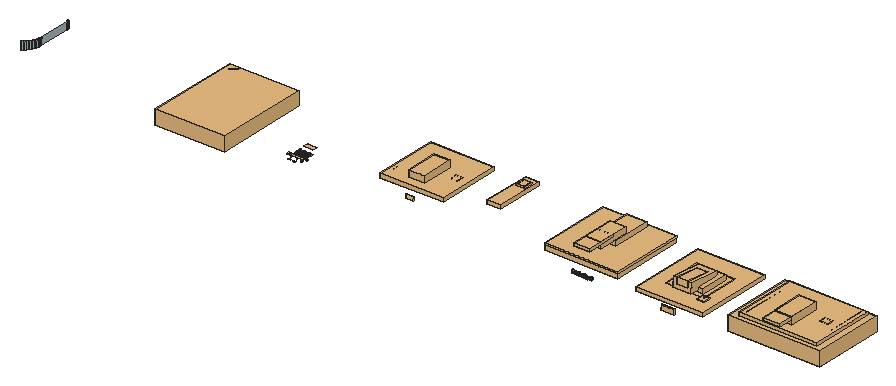
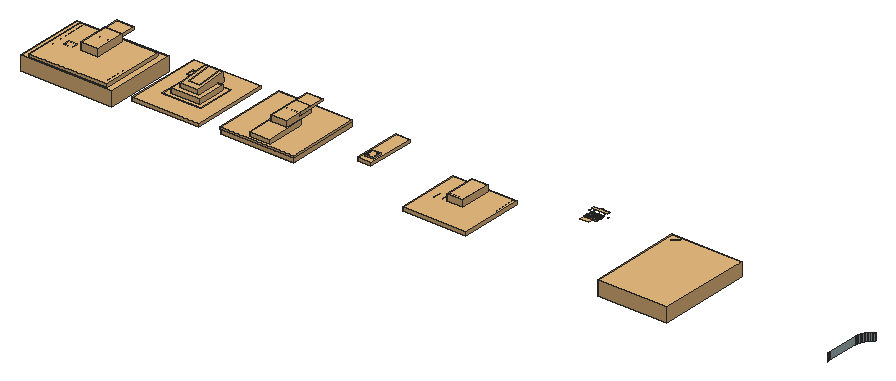
# SketchUp Ruby script. Lengths in inches.
U = 1.inch
M = Sketchup.active_model
def pt(a) = Geom::Point3d.new(a.map { |v| v * U })
def face(e, loops, mat)
  f = e.add_face(loops[0].map { |a| pt(a) })
  loops[1..].each { |l| e.add_face(l.map { |a| pt(a) }).erase! }
  f.material = f.back_material = mat if mat
  f
end
# faces: each face lists its corners as indices into pts; further lists are holes
def faces(e, pts, list, mat = nil) = list.each { |f| face(e, (f[0].is_a?(Array) ? f : [f]).map { |l| l.map { |i| pts[i] } }, mat) }
# xy, xz, yz: faces in a plane at the given z, y or x. An outline is a flat list of corners, or four numbers for a rectangle; further outlines are holes
def ring(l) = l.size == 4 ? [[l[0], l[1]], [l[2], l[1]], [l[2], l[3]], [l[0], l[3]]] : l.each_slice(2).to_a
def flat(e, list, mat, &to3) = list.each { |f| face(e, (f[0].is_a?(Array) ? f : [f]).map { |l| ring(l).map { |u, v| to3.(u, v) } }, mat) }
def xy(e, z, list, mat = nil) = flat(e, list, mat) { |x, y| [x, y, z] }
def xz(e, y, list, mat = nil) = flat(e, list, mat) { |x, z| [x, y, z] }
def yz(e, x, list, mat = nil) = flat(e, list, mat) { |y, z| [x, y, z] }
def lines(e, pts, list) = list.each { |a, b| e.add_line(pt(pts[a]), pt(pts[b])) }
# prism: a flat outline (further loops are holes) pulled along v
def prism(e, loops, v, mat = nil)
  f = face(e, loops, mat); d = Geom::Vector3d.new(v.map { |x| x * U })
  f.pushpull(f.normal.samedirection?(d) ? d.length : -d.length)
end
def box(e, o, s, mat = nil) = prism(e, [[o, [o[0] + s[0], o[1], o[2]], [o[0] + s[0], o[1] + s[1], o[2]], [o[0], o[1] + s[1], o[2]]]], [0, 0, s[2]], mat)
def at(x, y, z, deg = 0) = Geom::Transformation.translation(pt([x, y, z])) * Geom::Transformation.rotation(ORIGIN, Z_AXIS, deg.degrees)
def axes(o, x, y, z) = Geom::Transformation.new([*x, 0, *y, 0, *z, 0, *pt(o).to_a, 1])
def part(name) = M.definitions.add(name)
# library, detail: a bought-in or finely detailed component or shape, given as its bounding box
def library(name, o, s) = part(name).tap { |d| box(d.entities, o, s) }
def detail(e, o, s) = box(e.add_group.entities, o, s)
def put(e, d, t, mat = nil) = e.add_instance(d, t).tap { |i| i.material = mat if mat }
def group(e, t, mat = nil) = e.add_group.tap { |g| g.transformation = t; g.material = mat if mat }.entities
root = M.entities
M.materials.add("1").color = [0, 0, 0]
M.materials.add("11").color = [255, 255, 255]
M.materials.add("12").color = [5, 5, 5]
M.materials.add("2").color = [12, 12, 16]
M.materials.add("24").color = [74, 74, 74]
M.materials.add("26").color = [169, 186, 191]
M.materials.add("8").color = [50, 50, 50]
M.materials.add("9").color = [44, 44, 44]
c1 = library("Group89",[-140.11,-176.26,170.27],[282.52,381.26,57.85])
c2 = library("Group78",[38808.2,7300.17,1634.6875],[7.14,3.55,0.08])
c3 = library("Group72",[38808.13,7304.67,1634.69],[7.28,3.54,0.08])
c4 = library("Group73",[38807.56,7322.91,1634.71],[8.42,4.13,0.08])
c5 = library("om.cn_51",[-14089.91,-120000,166752.75],[16176.5,10000,4589.03])
c6 = library("om.cn_51698238",[-12277.97,-120000,175247.47],[24687.75,10000,11950.5])
c7 = library("Group79",[38826.73,7301.99,1634.69],[8.28,4.18,0.08])
c8 = library("Group74",[38826.7,7322.86,1634.71],[8.34,4.15,0.08])
c9 = library("om.cn_51268574",[-7425.4375,-120000,166763.1875],[21515.3125,10000,4564.15])
c10 = library("Group80",[38845.76,7302.01,1634.69],[8.44,4.16,0.08])
c11 = library("Group76",[38845.73,7322.86,1634.71],[8.5,4.18,0.08])
c12 = library("om.cn_32",[-31.33,-200.31,17.07],[62.68,126.37,27.34])
c13 = library("om.cn_32430148",[-31.33,-200.31,34.56],[62.68,118.17,8.93])
c14 = library("Group41",[2.42,129.72,-129.67],[259.34,15.26,259.34])
c15 = library("Group42",[13.39,138.09,-118.66],[237.39,3.26,237.32])
c16 = library("Group39",[-54.28,-6.65,-0.51],[57.5,23.32,1.99])
c17 = library("Group43",[197.75,140.28,-13.26],[27.5,3.46,26.52])
c18 = library("Group30",[-30.87,-113.18,-1.53],[61.73,214.81,14.15])
c19 = library("Group35",[-24.97,-25.2,0],[49.93,50.08,7.81])
c20 = library("Group16",[-41.15,-138.36,2.25],[82.3,160.65,19.68])
c21 = library("Group14",[-159,-159,0.16],[318,318,8.06])
c22 = library("Group13",[-149.91,-149.91,254.4375],[299.82,299.82,15.58])
c23 = library("Group46",[60.41,189.4,-65.28],[131.43,26.74,130.56])
c24 = library("Group53",[39.65,186.43,-85.24],[172.95,8.17,170.48])
c25 = library("Group54",[-24.48,177.31,-174.76],[301.22,16.77,349.52])
c26 = library("Group49",[134.43,190.47,6.48],[47.92,30.54,112.32])
c27 = library("Group55",[117.125,172.9375,-23.28],[82.52,48.07,142.08])
c28 = library("Group52",[-54.25,-6.65,-1.45],[57.46,23.32,2.82])
c29 = library("Group51",[197.5,187.71,76.61],[33.96,7.14,33.51])
c30 = library("Group5",[-32.86,-200.31,17.11],[65.72,126.37,27.3])
c31 = library("Group6",[-32.49,-200.31,34.57],[64.98,118.17,8.93])
c32 = library("Group7",[-18.29,129.75,-129.67],[300.75,15.26,259.34])
c33 = library("Group",[-44.84,79.83,-140.46],[353.86,54.36,289.99])
c34 = library("Group8",[40587.56,7377.77,1637.51],[284.38,237.38,4.11])
c35 = library("Group10",[40712.23,7354.21,1598.9],[39.27,4.15,12.57])
c36 = library("Group9",[206.09,140.95,-13.26],[31.34,3.18,26.52])
xy(root,91.8361,[[298.2685,7.251,298.2737,7.2799,298.2785,7.3089],[298.2785,7.3089,298.2831,7.3379,298.2873,7.367],[298.2873,7.367,298.2914,7.3965,298.2951,7.426],[298.2951,7.426,298.2985,7.4555,298.3017,7.4851],[298.3017,7.4851,298.3045,7.5147,298.3071,7.5443],
  [298.3092,12.9012,298.3071,12.9296,298.3045,12.9592],[298.3045,12.9592,298.3017,12.9888,298.2985,13.0184,298.2914,13.0775],[298.2985,13.0184,298.2951,13.048,298.2914,13.0775],[298.2914,13.0775,298.2873,13.107,298.2831,13.136]],"26")
xy(root,92.317,[[[384.7707,4.8659,390.0066,4.8659,390.2382,4.874,390.2707,4.8765,390.3033,4.8793,390.3357,4.8824,390.3682,4.8858,390.4006,4.8896,390.433,4.8937,390.4654,4.8981,390.4973,4.9028,390.5291,4.9078,390.5609,4.9131,390.5927,4.9188,390.6244,4.9248,390.656,4.931,390.6876,4.9376,390.9044,4.9919,391.1152,5.0606,391.3194,5.1429,391.5165,5.2385,391.7059,5.3467,391.8871,5.4669,392.0595,5.5987,392.2226,5.7415,392.3758,5.8947,392.5186,6.0578,392.6504,6.2302,392.7707,6.4114,392.8788,6.6008,392.9744,6.7979,393.0568,7.0021,393.1254,7.2129,393.1797,7.4297,393.1863,7.4613,393.1926,7.4929,393.1985,7.5246,393.2042,7.5564,393.2095,7.5882,393.2145,7.6201,393.2192,7.652,393.2236,7.6843,393.2277,7.7167,393.2315,7.7491,393.2349,7.7816,393.2381,7.8141,393.2408,7.8466,393.2433,7.8791,393.2515,8.1107,393.2515,13.3466,393.2433,13.5782,393.2408,13.6107,393.2381,13.6432,393.2349,13.6757,393.2315,13.7082,393.2277,13.7406,393.2236,13.773,393.2192,13.8053,393.2145,13.8372,393.2095,13.8691,393.2042,13.9009,393.1985,13.9327,393.1926,13.9644,393.1863,13.996,393.1797,14.0276,393.1254,14.2444,393.0568,14.4552,392.9744,14.6594,392.8788,14.8565,392.7707,15.0459,392.6504,15.2271,392.5186,15.3995,392.3758,15.5626,392.2226,15.7158,392.0595,15.8586,391.8871,15.9904,391.7059,16.1106,391.5165,16.2188,391.3194,16.3144,391.1152,16.3967,390.9044,16.4654,390.6876,16.5197,390.656,16.5263,390.6244,16.5326,390.5927,16.5385,390.5609,16.5442,390.5291,16.5495,390.4973,16.5545,390.4654,16.5592,390.433,16.5636,390.4006,16.5677,390.3682,16.5715,390.3357,16.5749,390.3033,16.578,390.2707,16.5808,390.2382,16.5833,390.0066,16.5914,384.7707,16.5914,384.5392,16.5833,384.5066,16.5808,384.4741,16.578,384.4416,16.5749,384.4091,16.5715,384.3767,16.5677,384.3443,16.5636,384.312,16.5592,384.2801,16.5545,384.2482,16.5495,384.2164,16.5442,384.1846,16.5385,384.1529,16.5326,384.1213,16.5263,384.0897,16.5197,383.8729,16.4654,383.6622,16.3967,383.458,16.3144,383.2609,16.2188,383.0715,16.1106,382.8903,15.9904,382.7178,15.8586,382.5548,15.7158,382.4015,15.5626,382.2588,15.3995,382.127,15.2271,382.0067,15.0459,381.8985,14.8565,381.803,14.6594,381.7206,14.4552,381.652,14.2444,381.5976,14.0276,381.5911,13.996,381.5848,13.9644,381.5788,13.9327,381.5732,13.9009,381.5678,13.8691,381.5628,13.8372,381.5581,13.8053,381.5537,13.773,381.5496,13.7406,381.5459,13.7082,381.5424,13.6757,381.5393,13.6432,381.5365,13.6107,381.534,13.5782,381.5259,13.3466,381.5259,8.1107,381.534,7.8791,381.5365,7.8466,381.5393,7.8141,381.5424,7.7816,381.5459,7.7491,381.5496,7.7167,381.5537,7.6843,381.5581,7.652,381.5628,7.6201,381.5678,7.5882,381.5732,7.5564,381.5788,7.5246,381.5848,7.4929,381.591,7.4613,381.5976,7.4297,381.652,7.2129,381.7206,7.0021,381.803,6.7979,381.8985,6.6008,382.0067,6.4114,382.127,6.2302,382.2588,6.0578,382.4015,5.8947,382.5548,5.7415,382.7178,5.5987,382.8903,5.4669,383.0714,5.3467,383.2609,5.2385,383.4579,5.1429,383.6622,5.0606,383.8729,4.9919,384.0897,4.9376,384.1213,4.931,384.1529,4.9248,384.1846,4.9188,384.2164,4.9131,384.2482,4.9078,384.2801,4.9028,384.312,4.8981,384.3443,4.8937,384.3767,4.8896,384.4091,4.8858,384.4416,4.8824,384.4741,4.8793,384.5066,4.8765,384.5392,4.874],[381.6833,7.4494,381.6772,7.4788,381.6711,7.5096,381.6653,7.5404,381.6598,7.5713,381.6498,7.6333,381.6452,7.6643,381.6409,7.6958,381.6369,7.7273,381.6332,7.7588,381.6299,7.7904,381.6269,7.822,381.6241,7.8537,381.6218,7.884,381.6269,7.822,381.6409,7.6958,381.6598,7.5713,381.6711,7.5096],[393.1555,13.5733,393.1505,13.6353,393.1364,13.7615,393.1175,13.886,393.1062,13.9477,393.094,14.0079,393.1001,13.9785,393.1062,13.9477,393.112,13.9169,393.1175,13.886,393.1276,13.824,393.1321,13.793,393.1364,13.7615,393.1404,13.73,393.1441,13.6985,393.1475,13.6669,393.1505,13.6353,393.1532,13.6036],[384.1094,16.434,384.1388,16.4401,384.1696,16.4462,384.2005,16.452,384.2314,16.4575,384.2933,16.4676,384.3243,16.4721,384.3558,16.4764,384.3873,16.4804,384.4189,16.4841,384.4504,16.4874,384.4821,16.4905,384.5137,16.4932,384.544,16.4955,384.4821,16.4905,384.3558,16.4764,384.2314,16.4575,384.1696,16.4462],[390.2333,4.9618,390.2953,4.9668,390.4216,4.9809,390.546,4.9998,390.6077,5.0111,390.6679,5.0233,390.6385,5.0172,390.6077,5.0111,390.5769,5.0053,390.546,4.9998,390.4841,4.9897,390.453,4.9852,390.4216,4.9809,390.39,4.9769,390.3585,4.9732,390.3269,4.9699,390.2953,4.9668,390.2637,4.9641],[393.112,7.5404,393.1227,7.6023,393.1321,7.6643,393.1404,7.7273,393.1475,7.7904,393.1532,7.8537,393.1505,7.822,393.1475,7.7904,393.1441,7.7588,393.1404,7.7273,393.1364,7.6958,393.1321,7.6643,393.1276,7.6333,393.1227,7.6023,393.1175,7.5713],[381.6241,13.6036,381.6269,13.6353,381.6299,13.6669,381.6332,13.6985,381.6369,13.73,381.6409,13.7615,381.6452,13.793,381.6498,13.824,381.6546,13.855,381.6598,13.886,381.6653,13.9169,381.6546,13.855,381.6452,13.793,381.6369,13.73,381.6299,13.6669],[390.5769,16.452,390.515,16.4627,390.453,16.4721,390.39,16.4804,390.3269,16.4874,390.2637,16.4932,390.2953,16.4905,390.3269,16.4874,390.3585,16.4841,390.39,16.4804,390.4216,16.4764,390.453,16.4721,390.4841,16.4676,390.515,16.4627,390.546,16.4575],[384.5137,4.9641,384.4821,4.9668,384.4504,4.9699,384.4189,4.9732,384.3873,4.9769,384.3558,4.9809,384.3243,4.9852,384.2933,4.9897,384.2623,4.9946,384.2314,4.9998,384.2005,5.0053,384.2623,4.9946,384.3243,4.9852,384.3873,4.9769,384.4504,4.9699]],[390.2333,4.9618,390.2637,4.9641,390.2953,4.9668],[384.5137,4.9641,384.4504,4.9699,384.4821,4.9668],[390.2953,4.9668,390.3269,4.9699,390.3585,4.9732,390.4216,4.9809],[384.4504,4.9699,384.3873,4.9769,384.4189,4.9732],
  [390.3585,4.9732,390.39,4.9769,390.4216,4.9809],[384.3873,4.9769,384.3243,4.9852,384.3558,4.9809],[390.4216,4.9809,390.453,4.9852,390.4841,4.9897],[390.4216,4.9809,390.4841,4.9897,390.546,4.9998],[384.3243,4.9852,384.2623,4.9946,384.2933,4.9897],
  [384.2623,4.9946,384.2005,5.0053,384.2314,4.9998],[390.546,4.9998,390.5769,5.0053,390.6077,5.0111],[390.6077,5.0111,390.6385,5.0172,390.6679,5.0233],[381.6833,7.4494,381.6711,7.5096,381.6772,7.4788],[381.6711,7.5096,381.6598,7.5713,381.6653,7.5404],
  [393.112,7.5404,393.1175,7.5713,393.1227,7.6023],[381.6598,7.5713,381.6409,7.6958,381.6498,7.6333],[393.1227,7.6023,393.1276,7.6333,393.1321,7.6643],[381.6498,7.6333,381.6409,7.6958,381.6452,7.6643],[393.1321,7.6643,393.1364,7.6958,393.1404,7.7273],
  [381.6409,7.6958,381.6269,7.822,381.6299,7.7904,381.6332,7.7588],[381.6409,7.6958,381.6332,7.7588,381.6369,7.7273],[393.1404,7.7273,393.1441,7.7588,393.1475,7.7904],[393.1475,7.7904,393.1505,7.822,393.1532,7.8537],[381.6269,7.822,381.6218,7.884,381.6241,7.8537]],"8")
yz(root,298.3991,[[7.7851,90.6622,12.6889,91.8361]],"26")
p = [[297.1213,5.309,90.6622],[297.1213,5.309,91.8361],[296.9516,5.1964,91.8361],[296.9516,5.1964,90.6622],[297.2827,5.4324,90.6622],[297.2827,5.4324,91.8361],
  [297.4355,5.5662,90.6622],[297.4355,5.5662,91.8361],[297.579,5.7097,90.6622],[297.579,5.7097,91.8361],[297.7127,5.8624,90.6622],[297.7127,5.8624,91.8361],
  [297.8361,6.0239,90.6622],[297.8361,6.0239,91.8361],[297.9488,6.1936,90.6622],[297.9488,6.1936,91.8361],[298.0501,6.371,90.6622],[298.0501,6.371,91.8361],
  [298.1396,6.5556,90.6622],[298.1396,6.5556,91.8361],[298.2167,6.7468,90.6622],[298.2167,6.7468,91.8361],[298.281,6.9442,90.6622],[298.281,6.9442,91.8361],
  [298.3319,7.1473,90.6622],[298.3319,7.1473,91.8361],[298.3381,7.1768,90.6622],[298.3381,7.1768,91.8361],[298.3439,7.2065,90.6622],[298.3439,7.2065,91.8361],
  [298.3495,7.2362,90.6622],[298.3495,7.2362,91.8361],[298.3548,7.2659,90.6622],[298.3548,7.2659,91.8361],[298.3598,7.2957,90.6622],[298.3598,7.2957,91.8361],
  [298.3645,7.3255,90.6622],[298.3645,7.3255,91.8361],[298.3689,7.3554,90.6622],[298.3689,7.3554,91.8361],[298.373,7.3857,90.6622],[298.373,7.3857,91.8361],
  [298.3768,7.4161,90.6622],[298.3768,7.4161,91.8361],[298.3804,7.4464,90.6622],[298.3804,7.4464,91.8361],[298.3836,7.4768,90.6622],[298.3836,7.4768,91.8361],
  [298.3865,7.5073,90.6622],[298.3865,7.5073,91.8361],[298.3891,7.5377,90.6622],[298.3891,7.5377,91.8361],[298.3914,7.5682,90.6622],[298.3914,7.5682,91.8361],
  [298.3991,7.7851,90.6622],[298.3991,7.7851,91.8361],[298.3915,12.9057,90.6622],[298.3915,12.9057,91.8361],[298.3991,12.6889,91.8361],[298.3991,12.6889,90.6622],
  [298.3865,12.9667,90.6622],[298.3865,12.9667,91.8361],[298.3891,12.9362,91.8361],[298.3891,12.9362,90.6622],[298.3768,13.0579,90.6622],[298.3768,13.0579,91.8361],
  [298.3804,13.0275,91.8361],[298.3804,13.0275,90.6622],[298.3836,12.9971,91.8361],[298.3836,12.9971,90.6622],[298.3689,13.1185,90.6622],[298.3689,13.1185,91.8361],
  [298.373,13.0882,91.8361],[298.373,13.0882,90.6622]]
faces(root,p,[[0,1,2,3],[4,5,1,0],[6,7,5,4],[8,9,7,6],[10,11,9,8],[12,13,11,10],[14,15,13,12],[16,17,15,14],
  [18,19,17,16],[20,21,19,18],[22,23,21,20],[24,25,23,22],[26,27,25,24],[28,29,27,26],[30,31,29,28],[32,33,31,30],
  [34,35,33,32],[36,37,35,34],[38,39,37,36],[40,41,39,38],[42,43,41,40],[44,45,43,42],[46,47,45,44],[48,49,47,46],
  [50,51,49,48],[52,53,51,50],[54,55,53,52],[56,57,58,59],[60,61,62,63],[63,62,57,56],[64,65,66,67],[67,66,68,69],
  [69,68,61,60],[70,71,72,73],[73,72,65,64]],"26")
g1 = group(root,at(326.82,8.82,83.09))
xy(g1,8.98,[[-2.48,-6.78,2.57,-6.78,3.23,-6.71,3.84,-6.49,4.375,-6.16,4.82,-5.72,5.16,-5.2,5.375,-4.61,5.45,-3.95,5.45,5.1,5.375,5.75,5.16,6.34,4.82,6.86,4.375,7.29,3.84,7.63,3.23,7.84,2.57,7.91,-2.48,7.91,-3.14,7.84,-3.75,7.63,-4.28,7.29,-4.73,6.86,-5.07,6.34,-5.28,5.75,-5.36,5.1,-5.36,-3.95,-5.28,-4.61,-5.07,-5.2,-4.73,-5.72,-4.28,-6.16,-3.75,-6.49,-3.14,-6.71]],"24")
put(root,c1,axes([326.82,8.82,83.09],[0.03937,0,0],[0,0.03937,0],[0,0,0.03937]))
g2 = group(root,at(-1185.85,-283.55,27.72))
detail(g2,[1527.72,287.27,64.36],[0.59,0.59,0.01])
g3 = group(root,at(-1185.85,-283.55,27.72))
detail(g3,[1527.72,288.09,64.36],[0.59,0.59,0.01])
put(root,c2,axes([-1185.85,-283.55,27.72],[0.03937,0,0],[0,0.03937,0],[0,0,0.03937]))
put(root,c3,axes([-1185.85,-283.55,27.72],[0.03937,0,0],[0,0.03937,0],[0,0,0.03937]))
put(root,c4,axes([-1185.85,-283.55,27.72],[0.03937,0,0],[0,0.03937,0],[0,0,0.03937]))
put(root,c5,axes([342.92,-12.12,92.39],[0.00009,0,0],[0,0,0],[0,0.00009,0]),"11")
g4 = group(root,at(342.92,-12.12,92.39))
prism(g4,[[[0.339,14.923,-0.339],[0.346,14.929,-0.339],[0.348,14.938,-0.339],[0.346,14.948,-0.339],[0.339,14.954,-0.339],[0.33,14.957,-0.339],[0.321,14.954,-0.339],[0.314,14.948,-0.339],[0.312,14.938,-0.339],[0.314,14.929,-0.339],[0.321,14.923,-0.339],[0.33,14.92,-0.339]]],[0,0,0.028],"11")
prism(g4,[[[-0.613,15.074,-0.339],[-0.61,15.084,-0.339],[-0.613,15.093,-0.339],[-0.619,15.099,-0.339],[-0.628,15.102,-0.339],[-0.638,15.099,-0.339],[-0.644,15.093,-0.339],[-0.647,15.084,-0.339],[-0.644,15.074,-0.339],[-0.638,15.068,-0.339],[-0.628,15.065,-0.339],[-0.619,15.068,-0.339]]],[0,0,0.028],"11")
prism(g4,[[[0.306,15.068,-0.339],[0.313,15.074,-0.339],[0.315,15.084,-0.339],[0.313,15.093,-0.339],[0.306,15.099,-0.339],[0.297,15.102,-0.339],[0.288,15.099,-0.339],[0.281,15.093,-0.339],[0.279,15.084,-0.339],[0.281,15.074,-0.339],[0.288,15.068,-0.339],[0.297,15.065,-0.339]]],[0,0,0.028],"11")
g5 = group(root,at(342.88,-15.8125,92.39))
box(g5,[-1.58,19.36,-0.34],[3.16,0.04,0.03],"11")
put(root,c6,axes([342.89,-4.82,92.39],[0.00006,0,0],[0,0,0],[0,0.00006,0]),"11")
g6 = group(root,at(-1185.85,-283.55,27.72))
detail(g6,[1528.47,287.27,64.36],[0.59,0.59,0.01])
g7 = group(root,at(-1185.85,-283.55,27.72))
detail(g7,[1528.47,288.09,64.36],[0.59,0.59,0.01])
g8 = group(root,at(342.92,-12.12,92.39))
prism(g8,[[[-0.624,14.471,-0.339],[0.624,14.471,-0.339],[0.629,14.473,-0.339],[0.632,14.476,-0.339],[0.633,14.48,-0.339],[0.633,14.516,-0.339],[0.632,14.521,-0.339],[0.629,14.524,-0.339],[0.624,14.525,-0.339],[-0.624,14.525,-0.339],[-0.629,14.524,-0.339],[-0.632,14.521,-0.339],[-0.633,14.516,-0.339],[-0.633,14.48,-0.339],[-0.632,14.476,-0.339],[-0.629,14.473,-0.339]]],[0,0,0.028],"11")
put(root,c7,axes([-1185.85,-283.55,27.72],[0.03937,0,0],[0,0.03937,0],[0,0,0.03937]))
put(root,c8,axes([-1185.85,-283.55,27.72],[0.03937,0,0],[0,0.03937,0],[0,0,0.03937]))
put(root,c9,axes([342.92,-12.12,92.39],[0.00009,0,0],[0,0,0],[0,0.00009,0]),"11")
g9 = group(root,at(-1185.85,-283.55,27.72))
detail(g9,[1529.22,287.27,64.36],[0.59,0.59,0.01])
g10 = group(root,at(-1185.85,-283.55,27.72))
detail(g10,[1529.22,288.09,64.36],[0.59,0.59,0.01])
put(root,c10,axes([-1185.85,-283.55,27.72],[0.03937,0,0],[0,0.03937,0],[0,0,0.03937]))
put(root,c11,axes([-1185.85,-283.55,27.72],[0.03937,0,0],[0,0.03937,0],[0,0,0.03937]))
g11 = group(root,at(342.92,-12.12,92.39))
prism(g11,[[[1.22,15.04,-0.34],[1.23,15.1,-0.34],[1.22,15.15,-0.34],[1.2,15.2,-0.34],[1.16,15.24,-0.34],[1.11,15.27,-0.34],[1.05,15.27,-0.34],[1,15.27,-0.34],[0.95,15.24,-0.34],[0.91,15.2,-0.34],[0.88,15.15,-0.34],[0.875,15.1,-0.34],[0.88,15.04,-0.34],[0.91,14.99,-0.34],[0.95,14.95,-0.34],[1,14.93,-0.34],[1.05,14.92,-0.34],[1.11,14.93,-0.34],[1.16,14.95,-0.34],[1.2,14.99,-0.34]],[[0.98,15.15,-0.34],[0.99,15.1,-0.34],[1.02,15.0625,-0.34],[1.05,15.03,-0.34],[1.1,15.02,-0.34],[1.14,15.02,-0.34],[1.1875,15.03,-0.34],[1.16,14.99,-0.34],[1.12,14.96,-0.34],[1.07,14.94,-0.34],[1.03,14.95,-0.34],[0.98,14.96,-0.34],[0.94,14.99,-0.34],[0.91,15.03,-0.34],[0.9,15.08,-0.34],[0.9,15.13,-0.34],[0.92,15.17,-0.34],[0.95,15.21,-0.34],[0.99,15.24,-0.34],[0.98,15.19,-0.34]]],[0,0,0.03],"11")
put(root,c12,axes([358.4,15.97,91.51],[0.03937,0,0],[0,0.03937,0],[0,0,0.03937]),"9")
put(root,c13,axes([358.4,15.97,91.51],[0.03937,0,0],[0,0.03937,0],[0,0,0.03937]),"2")
put(root,c14,axes([353.2,12.12,86.11],[0.03937,0,0],[0,0,0.03937],[0,-0.03937,0]))
put(root,c15,axes([353.2,11.9375,86.11],[0.03935,0.00137,0],[0,0,0.03937],[0.00137,-0.03935,0]))
put(root,c16,axes([359,6.6,90.23],[0.0209,0,0],[0,0.00397,0.02051],[0,-0.03687,0.00714]))
put(root,c17,axes([353.2,12.12,86.11],[0.03937,0,0],[0,0,0.03937],[0,-0.03937,0]))
put(root,c18,axes([371.95,10.64,93.87],[0.0359,-0.00031,0],[0.00031,0.0359,0],[0,0,0.0359]))
put(root,c19,axes([371.97,12.62,94.29],[0.02886,-0.00025,0],[0.00025,0.02886,0],[0,0,0.03231]))
g12 = group(root,at(371.99,12.62,94.4))
xy(g12,0,[[0.51,-0.53,-0.52,-0.52,-0.51,0.51,0.52,0.5]],"1")
xy(g12,0.06,[[0.51,-0.52,0.52,0.51,-0.51,0.52,-0.52,-0.51]],"1")
p = [[-0.51,0.52,0.06],[-0.51,0.51,0],[-0.52,-0.52,0],[-0.52,-0.51,0.06],[0.51,-0.53,0],[0.51,-0.52,0.06],
  [0.52,0.5,0],[0.52,0.51,0.06]]
faces(g12,p,[[0,1,2,3],[3,2,4,5],[5,4,6,7],[7,6,1,0]],"1")
put(root,c20,axes([387.3,15.29,92.4375],[0.03937,0,0],[0,0.03937,0],[0,0,0.03937]))
put(root,c12,axes([387.3,15.26,92.4375],[0.03937,0,0],[0,0.03937,0],[0,0,0.03937]),"8")
put(root,c13,axes([387.3,12.94,92.4375],[0.03937,0,0],[0,0.03937,0],[0,0,0.03937]),"8")
put(root,c21,axes([387.39,10.76,92.31],[0.03694,0,0],[0,0.03694,0],[0,0,0.04322]))
put(root,c22,axes([387.39,10.73,80.41],[0.03917,0,0],[0,0.03917,0],[0,0,0.04416]))
g13 = group(root,at(387.49,4.96,89.95))
box(g13,[-1.614,-0.158,0],[0.122,0.158,0.409],"12")
prism(g13,[[[-0.38,-0.158,0.174],[-0.38,-0.158,0.292],[-0.43,-0.158,0.292],[-0.43,-0.158,0.409],[-0.542,-0.158,0.409],[-0.542,-0.158,0.161],[-0.541,-0.158,0.139],[-0.539,-0.158,0.118],[-0.534,-0.158,0.099],[-0.528,-0.158,0.081],[-0.52,-0.158,0.065],[-0.51,-0.158,0.05],[-0.499,-0.158,0.037],[-0.486,-0.158,0.025],[-0.471,-0.158,0.016],[-0.455,-0.158,0.008],[-0.438,-0.158,0.001],[-0.419,-0.158,-0.003],[-0.399,-0.158,-0.006],[-0.378,-0.158,-0.007],[-0.378,-0.158,0.111],[-0.386,-0.158,0.111],[-0.393,-0.158,0.112],[-0.4,-0.158,0.114],[-0.406,-0.158,0.116],[-0.411,-0.158,0.118],[-0.415,-0.158,0.121],[-0.419,-0.158,0.125],[-0.422,-0.158,0.129],[-0.424,-0.158,0.134],[-0.426,-0.158,0.14],[-0.428,-0.158,0.147],[-0.429,-0.158,0.155],[-0.43,-0.158,0.164],[-0.43,-0.158,0.174]]],[0,0.158,0],"12")
prism(g13,[[[0.518,-0.158,0.174],[0.518,-0.158,0.292],[0.468,-0.158,0.292],[0.468,-0.158,0.409],[0.356,-0.158,0.409],[0.356,-0.158,0.161],[0.357,-0.158,0.139],[0.359,-0.158,0.118],[0.364,-0.158,0.099],[0.37,-0.158,0.081],[0.378,-0.158,0.065],[0.388,-0.158,0.05],[0.399,-0.158,0.037],[0.412,-0.158,0.025],[0.427,-0.158,0.016],[0.443,-0.158,0.008],[0.46,-0.158,0.001],[0.479,-0.158,-0.003],[0.499,-0.158,-0.006],[0.52,-0.158,-0.007],[0.52,-0.158,0.111],[0.512,-0.158,0.111],[0.505,-0.158,0.112],[0.498,-0.158,0.114],[0.492,-0.158,0.116],[0.487,-0.158,0.118],[0.483,-0.158,0.121],[0.479,-0.158,0.125],[0.476,-0.158,0.129],[0.474,-0.158,0.134],[0.472,-0.158,0.14],[0.47,-0.158,0.147],[0.469,-0.158,0.155],[0.468,-0.158,0.164],[0.468,-0.158,0.174]]],[0,0.158,0],"12")
prism(g13,[[[1.612,-0.158,0.174],[1.612,-0.158,0.292],[1.562,-0.158,0.292],[1.562,-0.158,0.409],[1.449,-0.158,0.409],[1.449,-0.158,0.161],[1.45,-0.158,0.139],[1.453,-0.158,0.118],[1.457,-0.158,0.099],[1.463,-0.158,0.081],[1.471,-0.158,0.065],[1.481,-0.158,0.05],[1.493,-0.158,0.037],[1.506,-0.158,0.025],[1.52,-0.158,0.016],[1.536,-0.158,0.008],[1.554,-0.158,0.001],[1.572,-0.158,-0.003],[1.592,-0.158,-0.006],[1.614,-0.158,-0.007],[1.614,-0.158,0.111],[1.606,-0.158,0.111],[1.598,-0.158,0.112],[1.591,-0.158,0.114],[1.586,-0.158,0.116],[1.58,-0.158,0.118],[1.576,-0.158,0.121],[1.573,-0.158,0.125],[1.57,-0.158,0.129],[1.567,-0.158,0.134],[1.565,-0.158,0.14],[1.564,-0.158,0.147],[1.5625,-0.158,0.155],[1.562,-0.158,0.164],[1.562,-0.158,0.174]]],[0,0.158,0],"12")
detail(g13,[-1.42,-0.16,0],[0.27,0.16,0.31])
detail(g13,[-1.09,-0.16,0],[0.27,0.16,0.31])
detail(g13,[-0.78,-0.16,0],[0.21,0.16,0.3])
detail(g13,[-0.34,-0.16,-0.01],[0.31,0.16,0.32])
detail(g13,[0.04,-0.16,0],[0.26,0.16,0.31])
detail(g13,[0.76,-0.16,-0.11],[0.31,0.16,0.42])
detail(g13,[1.1,-0.16,-0.01],[0.31,0.16,0.32])
put(root,c23,axes([397.57,10.42,85.8],[0.03558,0,0],[0,0,0.03166],[0,-0.03558,0]))
put(root,c24,axes([397.57,10.42,85.8],[0.03558,0,0],[0,0,0.03166],[0,-0.03558,0]))
put(root,c25,axes([397.57,10.42,85.8],[0.03558,0,0],[0,0,0.03166],[0,-0.03558,0]))
put(root,c26,axes([396.42,10.43,86.4],[0.03558,0,0],[0,0.00294,0.03152],[0,-0.03543,0.00331]))
put(root,c27,axes([396.42,10.43,86.4],[0.03558,0,0],[0,0.00294,0.03152],[0,-0.03543,0.00331]))
put(root,c28,axes([402.97,3.93,90.46],[0.03558,0,0],[0,0.0005,0.03558],[0,-0.03558,0.0005]))
put(root,c29,axes([397.57,10.42,85.8],[0.03558,0,0],[0,0,0.03166],[0,-0.03558,0]))
put(root,c30,axes([417.67,15.4375,92.15],[0.0415,0,0],[0,0.03937,0],[0,0,0.0415]))
put(root,c31,axes([417.67,13.11,92.15],[0.0415,0,0],[0,0.03937,0],[0,0,0.0415]))
put(root,c32,axes([412.2,11.58,86.46],[0.0415,0,0],[0,0,0.0415],[0,-0.03937,0]))
put(root,c33,axes([412.2,11.58,86.46],[0.0415,0,0],[0,0,0.0415],[0,-0.03937,0]))
put(root,c34,axes([-1185.85,-283.55,27.72],[0.03937,0,0],[0,0.03937,0],[0,0,0.03937]))
put(root,c35,axes([-1185.85,-283.55,27.72],[0.03937,0,0],[0,0.03937,0],[0,0,0.03937]))
put(root,c36,axes([412.2,11.58,86.46],[0.0415,0,0],[0,0,0.0415],[0,-0.03937,0]))
